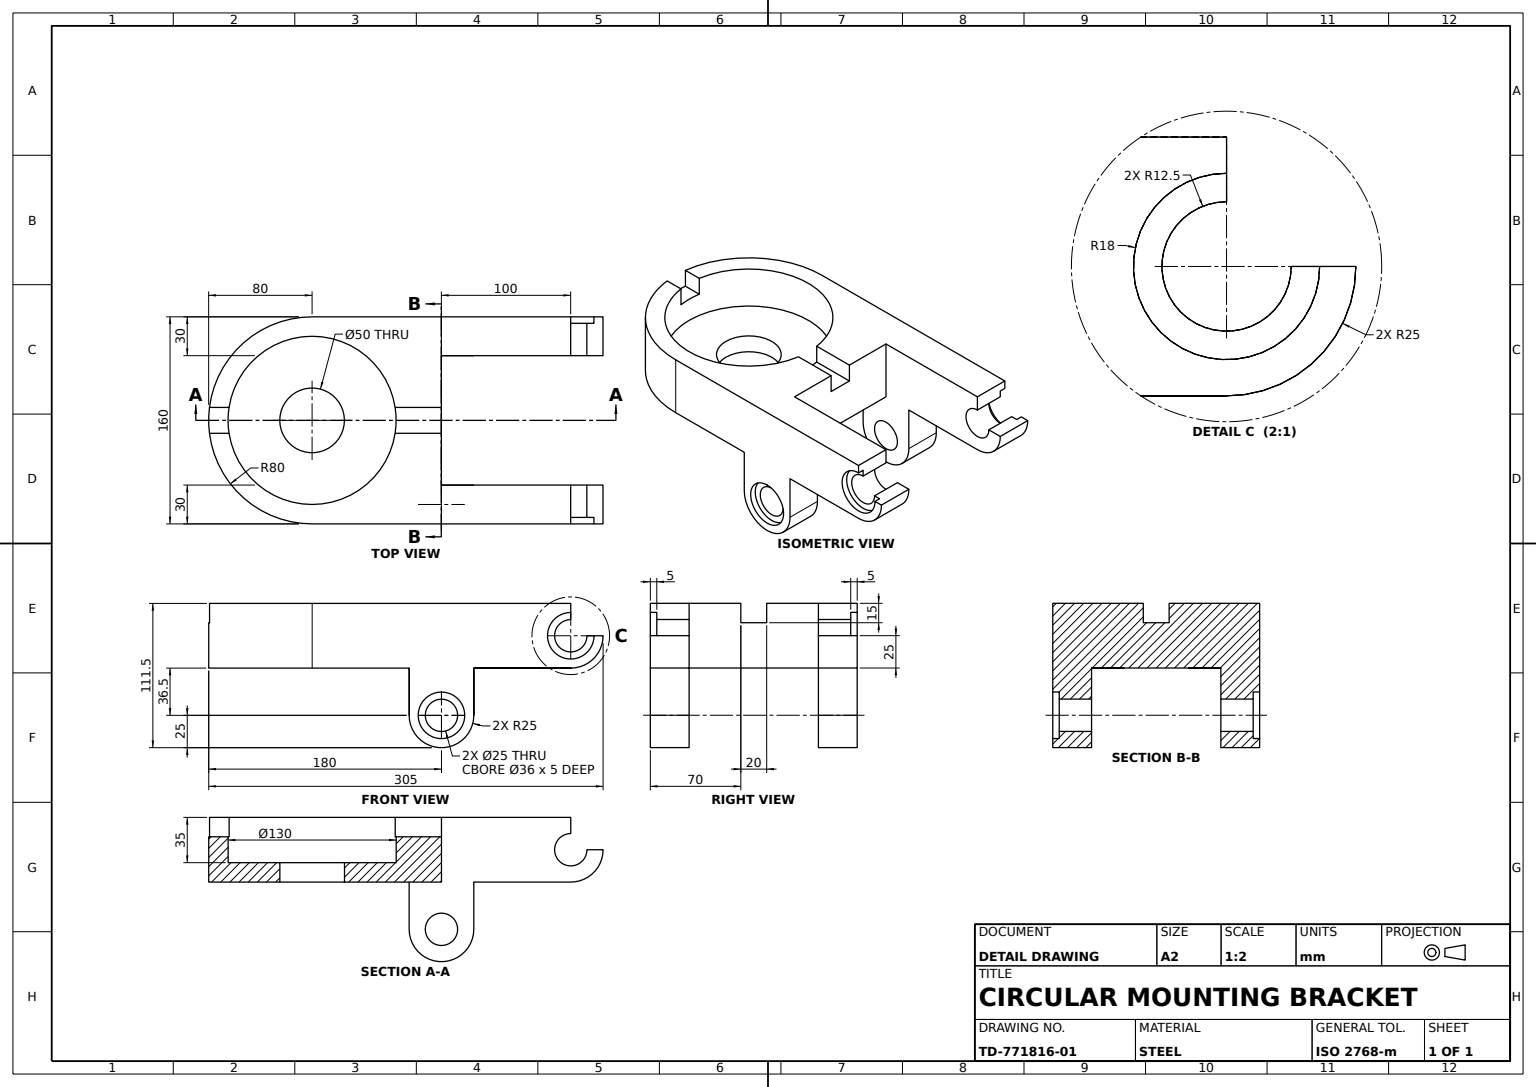
ISO-10303-21;
HEADER;
FILE_DESCRIPTION((''),'2;1');
FILE_NAME('','',(''),(''),'','','');
FILE_SCHEMA(('AUTOMOTIVE_DESIGN'));
ENDSEC;
DATA;
#1=APPLICATION_CONTEXT('');
#2=PRODUCT_CONTEXT('',#1,'mechanical');
#3=PRODUCT('','','',(#2));
#4=PRODUCT_DEFINITION_FORMATION('','',#3);
#5=PRODUCT_DEFINITION_CONTEXT('',#1,'design');
#6=PRODUCT_DEFINITION('','',#4,#5);
#7=PRODUCT_DEFINITION_SHAPE('','',#6);
#8=(LENGTH_UNIT()NAMED_UNIT(*)SI_UNIT(.MILLI.,.METRE.));
#9=(NAMED_UNIT(*)PLANE_ANGLE_UNIT()SI_UNIT($,.RADIAN.));
#10=(NAMED_UNIT(*)SI_UNIT($,.STERADIAN.)SOLID_ANGLE_UNIT());
#11=UNCERTAINTY_MEASURE_WITH_UNIT(LENGTH_MEASURE(0.005),#8,'distance_accuracy_value','');
#12=(GEOMETRIC_REPRESENTATION_CONTEXT(3)GLOBAL_UNCERTAINTY_ASSIGNED_CONTEXT((#11))GLOBAL_UNIT_ASSIGNED_CONTEXT((#8,#9,#10))REPRESENTATION_CONTEXT('',''));
#13=CARTESIAN_POINT('',(212.5,50.,25.));
#14=VERTEX_POINT('',#13);
#15=CARTESIAN_POINT('',(200.,50.,37.5));
#16=VERTEX_POINT('',#15);
#17=CARTESIAN_POINT('',(200.,50.,25.));
#18=DIRECTION('',(0.,1.,0.));
#19=DIRECTION('',(-1.,0.,0.));
#20=AXIS2_PLACEMENT_3D('',#17,#18,#19);
#21=CIRCLE('',#20,12.5);
#22=EDGE_CURVE('',#14,#16,#21,.T.);
#23=ORIENTED_EDGE('',*,*,#22,.F.);
#24=CARTESIAN_POINT('',(212.5,75.,25.));
#25=VERTEX_POINT('',#24);
#26=CARTESIAN_POINT('',(212.5,35.,25.));
#27=DIRECTION('',(0.,-1.,0.));
#28=VECTOR('',#27,1000.);
#29=LINE('',#26,#28);
#30=EDGE_CURVE('',#14,#25,#29,.F.);
#31=ORIENTED_EDGE('',*,*,#30,.T.);
#32=CARTESIAN_POINT('',(200.,75.,37.5));
#33=VERTEX_POINT('',#32);
#34=CARTESIAN_POINT('',(200.,75.,25.));
#35=DIRECTION('',(0.,0.,-1.));
#36=AXIS2_PLACEMENT_3D('',#34,#27,#35);
#37=CIRCLE('',#36,12.5);
#38=EDGE_CURVE('',#25,#33,#37,.F.);
#39=ORIENTED_EDGE('',*,*,#38,.T.);
#40=CARTESIAN_POINT('',(200.,35.,37.5));
#41=LINE('',#40,#28);
#42=EDGE_CURVE('',#33,#16,#41,.T.);
#43=ORIENTED_EDGE('',*,*,#42,.T.);
#44=EDGE_LOOP('',(#23,#31,#39,#43));
#45=FACE_BOUND('',#44,.T.);
#46=CARTESIAN_POINT('',(200.,35.,25.));
#47=AXIS2_PLACEMENT_3D('',#46,#27,#35);
#48=CYLINDRICAL_SURFACE('',#47,12.5);
#49=ADVANCED_FACE('',(#45),#48,.F.);
#50=CARTESIAN_POINT('',(100.,-10.,35.));
#51=VERTEX_POINT('',#50);
#52=CARTESIAN_POINT('',(100.,10.,35.));
#53=VERTEX_POINT('',#52);
#54=CARTESIAN_POINT('',(100.,-50.,35.));
#55=VECTOR('',#18,1000.);
#56=LINE('',#54,#55);
#57=EDGE_CURVE('',#51,#53,#56,.T.);
#58=ORIENTED_EDGE('',*,*,#57,.T.);
#59=CARTESIAN_POINT('',(64.226163,10.,35.));
#60=VERTEX_POINT('',#59);
#61=CARTESIAN_POINT('',(115.961249,10.,35.));
#62=VECTOR('',#19,1000.);
#63=LINE('',#61,#62);
#64=EDGE_CURVE('',#60,#53,#63,.F.);
#65=ORIENTED_EDGE('',*,*,#64,.F.);
#66=CARTESIAN_POINT('',(64.226163,-10.,35.));
#67=VERTEX_POINT('',#66);
#68=CARTESIAN_POINT('',(0.,0.,35.));
#69=DIRECTION('',(0.,0.,1.));
#70=DIRECTION('',(1.,0.,0.));
#71=AXIS2_PLACEMENT_3D('',#68,#69,#70);
#72=CIRCLE('',#71,65.);
#73=EDGE_CURVE('',#60,#67,#72,.F.);
#74=ORIENTED_EDGE('',*,*,#73,.T.);
#75=CARTESIAN_POINT('',(-115.961249,-10.,35.));
#76=VECTOR('',#70,1000.);
#77=LINE('',#75,#76);
#78=EDGE_CURVE('',#51,#67,#77,.F.);
#79=ORIENTED_EDGE('',*,*,#78,.F.);
#80=EDGE_LOOP('',(#58,#65,#74,#79));
#81=FACE_BOUND('',#80,.T.);
#82=PLANE('',#71);
#83=ADVANCED_FACE('',(#81),#82,.T.);
#84=CARTESIAN_POINT('',(200.,-80.,0.));
#85=VERTEX_POINT('',#84);
#86=CARTESIAN_POINT('',(125.,-80.,0.));
#87=VERTEX_POINT('',#86);
#88=CARTESIAN_POINT('',(100.,-80.,0.));
#89=LINE('',#88,#62);
#90=EDGE_CURVE('',#85,#87,#89,.T.);
#91=ORIENTED_EDGE('',*,*,#90,.F.);
#92=CARTESIAN_POINT('',(225.,-80.,25.));
#93=VERTEX_POINT('',#92);
#94=CARTESIAN_POINT('',(200.,-80.,25.));
#95=AXIS2_PLACEMENT_3D('',#94,#27,#70);
#96=CIRCLE('',#95,25.);
#97=EDGE_CURVE('',#85,#93,#96,.T.);
#98=ORIENTED_EDGE('',*,*,#97,.T.);
#99=CARTESIAN_POINT('',(218.,-80.,25.));
#100=VERTEX_POINT('',#99);
#101=CARTESIAN_POINT('',(100.,-80.,25.));
#102=LINE('',#101,#76);
#103=EDGE_CURVE('',#100,#93,#102,.T.);
#104=ORIENTED_EDGE('',*,*,#103,.F.);
#105=CARTESIAN_POINT('',(200.,-80.,43.));
#106=VERTEX_POINT('',#105);
#107=AXIS2_PLACEMENT_3D('',#94,#18,#69);
#108=CIRCLE('',#107,18.);
#109=EDGE_CURVE('',#100,#106,#108,.T.);
#110=ORIENTED_EDGE('',*,*,#109,.T.);
#111=CARTESIAN_POINT('',(200.,-80.,50.));
#112=VERTEX_POINT('',#111);
#113=VECTOR('',#35,1000.);
#114=LINE('',#111,#113);
#115=EDGE_CURVE('',#112,#106,#114,.T.);
#116=ORIENTED_EDGE('',*,*,#115,.F.);
#117=CARTESIAN_POINT('',(0.,-80.,50.));
#118=VERTEX_POINT('',#117);
#119=CARTESIAN_POINT('',(100.,-80.,50.));
#120=LINE('',#119,#62);
#121=EDGE_CURVE('',#112,#118,#120,.T.);
#122=ORIENTED_EDGE('',*,*,#121,.T.);
#123=CARTESIAN_POINT('',(0.,-80.,0.));
#124=VERTEX_POINT('',#123);
#125=LINE('',#117,#113);
#126=EDGE_CURVE('',#118,#124,#125,.T.);
#127=ORIENTED_EDGE('',*,*,#126,.T.);
#128=CARTESIAN_POINT('',(75.,-80.,0.));
#129=VERTEX_POINT('',#128);
#130=EDGE_CURVE('',#129,#124,#89,.T.);
#131=ORIENTED_EDGE('',*,*,#130,.F.);
#132=CARTESIAN_POINT('',(75.,-80.,-36.5));
#133=VERTEX_POINT('',#132);
#134=CARTESIAN_POINT('',(75.,-80.,24.));
#135=LINE('',#134,#113);
#136=EDGE_CURVE('',#129,#133,#135,.T.);
#137=ORIENTED_EDGE('',*,*,#136,.T.);
#138=CARTESIAN_POINT('',(125.,-80.,-36.5));
#139=VERTEX_POINT('',#138);
#140=CARTESIAN_POINT('',(100.,-80.,-36.5));
#141=AXIS2_PLACEMENT_3D('',#140,#27,#70);
#142=CIRCLE('',#141,25.);
#143=EDGE_CURVE('',#133,#139,#142,.T.);
#144=ORIENTED_EDGE('',*,*,#143,.T.);
#145=VECTOR('',#69,1000.);
#146=LINE('',#138,#145);
#147=EDGE_CURVE('',#139,#87,#146,.T.);
#148=ORIENTED_EDGE('',*,*,#147,.T.);
#149=EDGE_LOOP('',(#91,#98,#104,#110,#116,#122,#127,#131,#137,#144,#148));
#150=FACE_BOUND('',#149,.T.);
#151=CARTESIAN_POINT('',(100.,-80.,-18.5));
#152=VERTEX_POINT('',#151);
#153=AXIS2_PLACEMENT_3D('',#140,#18,#69);
#154=CIRCLE('',#153,18.);
#155=EDGE_CURVE('',#152,#152,#154,.T.);
#156=ORIENTED_EDGE('',*,*,#155,.T.);
#157=EDGE_LOOP('',(#156));
#158=FACE_BOUND('',#157,.T.);
#159=AXIS2_PLACEMENT_3D('',#119,#27,#35);
#160=PLANE('',#159);
#161=ADVANCED_FACE('',(#150,#158),#160,.T.);
#162=CARTESIAN_POINT('',(75.,80.,0.));
#163=VERTEX_POINT('',#162);
#164=CARTESIAN_POINT('',(75.,80.,-36.5));
#165=VERTEX_POINT('',#164);
#166=CARTESIAN_POINT('',(75.,80.,24.));
#167=LINE('',#166,#113);
#168=EDGE_CURVE('',#163,#165,#167,.T.);
#169=ORIENTED_EDGE('',*,*,#168,.T.);
#170=CARTESIAN_POINT('',(75.,50.,-36.5));
#171=VERTEX_POINT('',#170);
#172=LINE('',#164,#28);
#173=EDGE_CURVE('',#165,#171,#172,.T.);
#174=ORIENTED_EDGE('',*,*,#173,.T.);
#175=CARTESIAN_POINT('',(75.,50.,0.));
#176=VERTEX_POINT('',#175);
#177=CARTESIAN_POINT('',(75.,50.,24.));
#178=LINE('',#177,#113);
#179=EDGE_CURVE('',#176,#171,#178,.T.);
#180=ORIENTED_EDGE('',*,*,#179,.F.);
#181=CARTESIAN_POINT('',(75.,0.,0.));
#182=LINE('',#181,#55);
#183=EDGE_CURVE('',#176,#163,#182,.T.);
#184=ORIENTED_EDGE('',*,*,#183,.T.);
#185=EDGE_LOOP('',(#169,#174,#180,#184));
#186=FACE_BOUND('',#185,.T.);
#187=AXIS2_PLACEMENT_3D('',#166,#19,#69);
#188=PLANE('',#187);
#189=ADVANCED_FACE('',(#186),#188,.T.);
#190=CARTESIAN_POINT('',(112.5,-50.,-36.5));
#191=VERTEX_POINT('',#190);
#192=CARTESIAN_POINT('',(100.,-50.,-36.5));
#193=AXIS2_PLACEMENT_3D('',#192,#27,#70);
#194=CIRCLE('',#193,12.5);
#195=EDGE_CURVE('',#191,#191,#194,.T.);
#196=ORIENTED_EDGE('',*,*,#195,.T.);
#197=EDGE_LOOP('',(#196));
#198=FACE_BOUND('',#197,.T.);
#199=CARTESIAN_POINT('',(75.,-50.,0.));
#200=VERTEX_POINT('',#199);
#201=CARTESIAN_POINT('',(100.,-50.,0.));
#202=VERTEX_POINT('',#201);
#203=CARTESIAN_POINT('',(0.,-50.,0.));
#204=LINE('',#203,#62);
#205=EDGE_CURVE('',#200,#202,#204,.F.);
#206=ORIENTED_EDGE('',*,*,#205,.T.);
#207=CARTESIAN_POINT('',(100.,-50.,50.));
#208=VERTEX_POINT('',#207);
#209=CARTESIAN_POINT('',(100.,-50.,120.));
#210=LINE('',#209,#113);
#211=EDGE_CURVE('',#202,#208,#210,.F.);
#212=ORIENTED_EDGE('',*,*,#211,.T.);
#213=CARTESIAN_POINT('',(200.,-50.,50.));
#214=VERTEX_POINT('',#213);
#215=CARTESIAN_POINT('',(0.,-50.,50.));
#216=LINE('',#215,#62);
#217=EDGE_CURVE('',#214,#208,#216,.T.);
#218=ORIENTED_EDGE('',*,*,#217,.F.);
#219=CARTESIAN_POINT('',(200.,-50.,37.5));
#220=VERTEX_POINT('',#219);
#221=CARTESIAN_POINT('',(200.,-50.,120.));
#222=LINE('',#221,#113);
#223=EDGE_CURVE('',#214,#220,#222,.T.);
#224=ORIENTED_EDGE('',*,*,#223,.T.);
#225=CARTESIAN_POINT('',(212.5,-50.,25.));
#226=VERTEX_POINT('',#225);
#227=CARTESIAN_POINT('',(200.,-50.,25.));
#228=AXIS2_PLACEMENT_3D('',#227,#27,#70);
#229=CIRCLE('',#228,12.5);
#230=EDGE_CURVE('',#220,#226,#229,.T.);
#231=ORIENTED_EDGE('',*,*,#230,.T.);
#232=CARTESIAN_POINT('',(225.,-50.,25.));
#233=VERTEX_POINT('',#232);
#234=CARTESIAN_POINT('',(220.,-50.,25.));
#235=LINE('',#234,#76);
#236=EDGE_CURVE('',#226,#233,#235,.T.);
#237=ORIENTED_EDGE('',*,*,#236,.T.);
#238=CARTESIAN_POINT('',(200.,-50.,0.));
#239=VERTEX_POINT('',#238);
#240=CIRCLE('',#228,25.);
#241=EDGE_CURVE('',#239,#233,#240,.T.);
#242=ORIENTED_EDGE('',*,*,#241,.F.);
#243=CARTESIAN_POINT('',(125.,-50.,0.));
#244=VERTEX_POINT('',#243);
#245=EDGE_CURVE('',#239,#244,#204,.T.);
#246=ORIENTED_EDGE('',*,*,#245,.T.);
#247=CARTESIAN_POINT('',(125.,-50.,-36.5));
#248=VERTEX_POINT('',#247);
#249=LINE('',#247,#145);
#250=EDGE_CURVE('',#248,#244,#249,.T.);
#251=ORIENTED_EDGE('',*,*,#250,.F.);
#252=CARTESIAN_POINT('',(75.,-50.,-36.5));
#253=VERTEX_POINT('',#252);
#254=CIRCLE('',#193,25.);
#255=EDGE_CURVE('',#253,#248,#254,.T.);
#256=ORIENTED_EDGE('',*,*,#255,.F.);
#257=CARTESIAN_POINT('',(75.,-50.,24.));
#258=LINE('',#257,#113);
#259=EDGE_CURVE('',#200,#253,#258,.T.);
#260=ORIENTED_EDGE('',*,*,#259,.F.);
#261=EDGE_LOOP('',(#206,#212,#218,#224,#231,#237,#242,#246,#251,#256,#260));
#262=FACE_BOUND('',#261,.T.);
#263=CARTESIAN_POINT('',(220.,-50.,120.));
#264=AXIS2_PLACEMENT_3D('',#263,#27,#70);
#265=PLANE('',#264);
#266=ADVANCED_FACE('',(#198,#262),#265,.F.);
#267=CARTESIAN_POINT('',(-79.372539,10.,35.));
#268=VERTEX_POINT('',#267);
#269=CARTESIAN_POINT('',(-64.226163,10.,35.));
#270=VERTEX_POINT('',#269);
#271=EDGE_CURVE('',#268,#270,#63,.F.);
#272=ORIENTED_EDGE('',*,*,#271,.F.);
#273=CARTESIAN_POINT('',(-79.372539,-10.,35.));
#274=VERTEX_POINT('',#273);
#275=CIRCLE('',#71,80.);
#276=EDGE_CURVE('',#274,#268,#275,.F.);
#277=ORIENTED_EDGE('',*,*,#276,.F.);
#278=CARTESIAN_POINT('',(-64.226163,-10.,35.));
#279=VERTEX_POINT('',#278);
#280=EDGE_CURVE('',#279,#274,#77,.F.);
#281=ORIENTED_EDGE('',*,*,#280,.F.);
#282=EDGE_CURVE('',#279,#270,#72,.F.);
#283=ORIENTED_EDGE('',*,*,#282,.T.);
#284=EDGE_LOOP('',(#272,#277,#281,#283));
#285=FACE_BOUND('',#284,.T.);
#286=ADVANCED_FACE('',(#285),#82,.T.);
#287=ORIENTED_EDGE('',*,*,#250,.T.);
#288=CARTESIAN_POINT('',(125.,0.,0.));
#289=LINE('',#288,#55);
#290=EDGE_CURVE('',#87,#244,#289,.T.);
#291=ORIENTED_EDGE('',*,*,#290,.F.);
#292=ORIENTED_EDGE('',*,*,#147,.F.);
#293=LINE('',#138,#55);
#294=EDGE_CURVE('',#139,#248,#293,.T.);
#295=ORIENTED_EDGE('',*,*,#294,.T.);
#296=EDGE_LOOP('',(#287,#291,#292,#295));
#297=FACE_BOUND('',#296,.T.);
#298=AXIS2_PLACEMENT_3D('',#138,#19,#69);
#299=PLANE('',#298);
#300=ADVANCED_FACE('',(#297),#299,.F.);
#301=CARTESIAN_POINT('',(100.,-75.,-24.));
#302=VERTEX_POINT('',#301);
#303=CARTESIAN_POINT('',(100.,-75.,-36.5));
#304=AXIS2_PLACEMENT_3D('',#303,#18,#69);
#305=CIRCLE('',#304,12.5);
#306=EDGE_CURVE('',#302,#302,#305,.F.);
#307=ORIENTED_EDGE('',*,*,#306,.F.);
#308=EDGE_LOOP('',(#307));
#309=FACE_BOUND('',#308,.T.);
#310=CARTESIAN_POINT('',(100.,-75.,-18.5));
#311=VERTEX_POINT('',#310);
#312=CIRCLE('',#304,18.);
#313=EDGE_CURVE('',#311,#311,#312,.F.);
#314=ORIENTED_EDGE('',*,*,#313,.T.);
#315=EDGE_LOOP('',(#314));
#316=FACE_BOUND('',#315,.T.);
#317=PLANE('',#304);
#318=ADVANCED_FACE('',(#309,#316),#317,.F.);
#319=CARTESIAN_POINT('',(-64.226163,10.,50.));
#320=VERTEX_POINT('',#319);
#321=CARTESIAN_POINT('',(-79.372539,10.,50.));
#322=VERTEX_POINT('',#321);
#323=CARTESIAN_POINT('',(0.,10.,50.));
#324=LINE('',#323,#62);
#325=EDGE_CURVE('',#320,#322,#324,.T.);
#326=ORIENTED_EDGE('',*,*,#325,.T.);
#327=LINE('',#321,#113);
#328=EDGE_CURVE('',#268,#322,#327,.F.);
#329=ORIENTED_EDGE('',*,*,#328,.F.);
#330=ORIENTED_EDGE('',*,*,#271,.T.);
#331=LINE('',#319,#113);
#332=EDGE_CURVE('',#270,#320,#331,.F.);
#333=ORIENTED_EDGE('',*,*,#332,.T.);
#334=EDGE_LOOP('',(#326,#329,#330,#333));
#335=FACE_BOUND('',#334,.T.);
#336=CARTESIAN_POINT('',(115.961249,10.,62.));
#337=AXIS2_PLACEMENT_3D('',#336,#27,#70);
#338=PLANE('',#337);
#339=ADVANCED_FACE('',(#335),#338,.T.);
#340=ORIENTED_EDGE('',*,*,#195,.F.);
#341=EDGE_LOOP('',(#340));
#342=FACE_BOUND('',#341,.T.);
#343=ORIENTED_EDGE('',*,*,#306,.T.);
#344=EDGE_LOOP('',(#343));
#345=FACE_BOUND('',#344,.T.);
#346=CARTESIAN_POINT('',(100.,-35.,-36.5));
#347=AXIS2_PLACEMENT_3D('',#346,#18,#69);
#348=CYLINDRICAL_SURFACE('',#347,12.5);
#349=ADVANCED_FACE('',(#342,#345),#348,.F.);
#350=CARTESIAN_POINT('',(200.,-75.,43.));
#351=VERTEX_POINT('',#350);
#352=LINE('',#105,#55);
#353=EDGE_CURVE('',#351,#106,#352,.F.);
#354=ORIENTED_EDGE('',*,*,#353,.T.);
#355=ORIENTED_EDGE('',*,*,#109,.F.);
#356=CARTESIAN_POINT('',(218.,-75.,25.));
#357=VERTEX_POINT('',#356);
#358=LINE('',#99,#55);
#359=EDGE_CURVE('',#100,#357,#358,.T.);
#360=ORIENTED_EDGE('',*,*,#359,.T.);
#361=CARTESIAN_POINT('',(200.,-75.,25.));
#362=AXIS2_PLACEMENT_3D('',#361,#18,#69);
#363=CIRCLE('',#362,18.);
#364=EDGE_CURVE('',#351,#357,#363,.F.);
#365=ORIENTED_EDGE('',*,*,#364,.F.);
#366=EDGE_LOOP('',(#354,#355,#360,#365));
#367=FACE_BOUND('',#366,.T.);
#368=CYLINDRICAL_SURFACE('',#107,18.);
#369=ADVANCED_FACE('',(#367),#368,.F.);
#370=CARTESIAN_POINT('',(212.5,-75.,25.));
#371=VERTEX_POINT('',#370);
#372=LINE('',#361,#62);
#373=EDGE_CURVE('',#357,#371,#372,.T.);
#374=ORIENTED_EDGE('',*,*,#373,.T.);
#375=CARTESIAN_POINT('',(200.,-75.,37.5));
#376=VERTEX_POINT('',#375);
#377=CIRCLE('',#362,12.5);
#378=EDGE_CURVE('',#376,#371,#377,.F.);
#379=ORIENTED_EDGE('',*,*,#378,.F.);
#380=LINE('',#361,#145);
#381=EDGE_CURVE('',#376,#351,#380,.T.);
#382=ORIENTED_EDGE('',*,*,#381,.T.);
#383=ORIENTED_EDGE('',*,*,#364,.T.);
#384=EDGE_LOOP('',(#374,#379,#382,#383));
#385=FACE_BOUND('',#384,.T.);
#386=PLANE('',#362);
#387=ADVANCED_FACE('',(#385),#386,.F.);
#388=CARTESIAN_POINT('',(218.,75.,25.));
#389=VERTEX_POINT('',#388);
#390=LINE('',#34,#76);
#391=EDGE_CURVE('',#25,#389,#390,.T.);
#392=ORIENTED_EDGE('',*,*,#391,.F.);
#393=ORIENTED_EDGE('',*,*,#30,.F.);
#394=CARTESIAN_POINT('',(225.,50.,25.));
#395=VERTEX_POINT('',#394);
#396=CARTESIAN_POINT('',(100.,50.,25.));
#397=LINE('',#396,#62);
#398=EDGE_CURVE('',#395,#14,#397,.T.);
#399=ORIENTED_EDGE('',*,*,#398,.F.);
#400=CARTESIAN_POINT('',(225.,80.,25.));
#401=VERTEX_POINT('',#400);
#402=LINE('',#400,#28);
#403=EDGE_CURVE('',#395,#401,#402,.F.);
#404=ORIENTED_EDGE('',*,*,#403,.T.);
#405=CARTESIAN_POINT('',(218.,80.,25.));
#406=VERTEX_POINT('',#405);
#407=CARTESIAN_POINT('',(0.,80.,25.));
#408=LINE('',#407,#62);
#409=EDGE_CURVE('',#401,#406,#408,.T.);
#410=ORIENTED_EDGE('',*,*,#409,.T.);
#411=LINE('',#405,#28);
#412=EDGE_CURVE('',#389,#406,#411,.F.);
#413=ORIENTED_EDGE('',*,*,#412,.F.);
#414=EDGE_LOOP('',(#392,#393,#399,#404,#410,#413));
#415=FACE_BOUND('',#414,.T.);
#416=CARTESIAN_POINT('',(232.692308,-110.,25.));
#417=AXIS2_PLACEMENT_3D('',#416,#35,#19);
#418=PLANE('',#417);
#419=ADVANCED_FACE('',(#415),#418,.F.);
#420=CARTESIAN_POINT('',(125.,80.,0.));
#421=VERTEX_POINT('',#420);
#422=CARTESIAN_POINT('',(125.,50.,0.));
#423=VERTEX_POINT('',#422);
#424=LINE('',#288,#28);
#425=EDGE_CURVE('',#421,#423,#424,.T.);
#426=ORIENTED_EDGE('',*,*,#425,.T.);
#427=CARTESIAN_POINT('',(125.,50.,-36.5));
#428=VERTEX_POINT('',#427);
#429=LINE('',#427,#145);
#430=EDGE_CURVE('',#428,#423,#429,.T.);
#431=ORIENTED_EDGE('',*,*,#430,.F.);
#432=CARTESIAN_POINT('',(125.,80.,-36.5));
#433=VERTEX_POINT('',#432);
#434=LINE('',#432,#28);
#435=EDGE_CURVE('',#433,#428,#434,.T.);
#436=ORIENTED_EDGE('',*,*,#435,.F.);
#437=LINE('',#432,#145);
#438=EDGE_CURVE('',#433,#421,#437,.T.);
#439=ORIENTED_EDGE('',*,*,#438,.T.);
#440=EDGE_LOOP('',(#426,#431,#436,#439));
#441=FACE_BOUND('',#440,.T.);
#442=AXIS2_PLACEMENT_3D('',#432,#70,#35);
#443=PLANE('',#442);
#444=ADVANCED_FACE('',(#441),#443,.T.);
#445=CARTESIAN_POINT('',(100.,80.,-54.5));
#446=VERTEX_POINT('',#445);
#447=CARTESIAN_POINT('',(100.,80.,-36.5));
#448=AXIS2_PLACEMENT_3D('',#447,#27,#35);
#449=CIRCLE('',#448,18.);
#450=EDGE_CURVE('',#446,#446,#449,.T.);
#451=ORIENTED_EDGE('',*,*,#450,.F.);
#452=EDGE_LOOP('',(#451));
#453=FACE_BOUND('',#452,.T.);
#454=CARTESIAN_POINT('',(100.,75.,-54.5));
#455=VERTEX_POINT('',#454);
#456=CARTESIAN_POINT('',(100.,75.,-36.5));
#457=AXIS2_PLACEMENT_3D('',#456,#27,#35);
#458=CIRCLE('',#457,18.);
#459=EDGE_CURVE('',#455,#455,#458,.F.);
#460=ORIENTED_EDGE('',*,*,#459,.F.);
#461=EDGE_LOOP('',(#460));
#462=FACE_BOUND('',#461,.T.);
#463=CYLINDRICAL_SURFACE('',#448,18.);
#464=ADVANCED_FACE('',(#453,#462),#463,.F.);
#465=ORIENTED_EDGE('',*,*,#328,.T.);
#466=CARTESIAN_POINT('',(0.,80.,50.));
#467=VERTEX_POINT('',#466);
#468=CARTESIAN_POINT('',(0.,0.,50.));
#469=AXIS2_PLACEMENT_3D('',#468,#35,#70);
#470=CIRCLE('',#469,80.);
#471=EDGE_CURVE('',#322,#467,#470,.T.);
#472=ORIENTED_EDGE('',*,*,#471,.T.);
#473=CARTESIAN_POINT('',(0.,80.,0.));
#474=VERTEX_POINT('',#473);
#475=LINE('',#466,#113);
#476=EDGE_CURVE('',#467,#474,#475,.T.);
#477=ORIENTED_EDGE('',*,*,#476,.T.);
#478=CARTESIAN_POINT('',(0.,0.,0.));
#479=AXIS2_PLACEMENT_3D('',#478,#35,#70);
#480=CIRCLE('',#479,80.);
#481=EDGE_CURVE('',#124,#474,#480,.T.);
#482=ORIENTED_EDGE('',*,*,#481,.F.);
#483=ORIENTED_EDGE('',*,*,#126,.F.);
#484=CARTESIAN_POINT('',(-79.372539,-10.,50.));
#485=VERTEX_POINT('',#484);
#486=EDGE_CURVE('',#118,#485,#470,.T.);
#487=ORIENTED_EDGE('',*,*,#486,.T.);
#488=LINE('',#484,#113);
#489=EDGE_CURVE('',#485,#274,#488,.T.);
#490=ORIENTED_EDGE('',*,*,#489,.T.);
#491=ORIENTED_EDGE('',*,*,#276,.T.);
#492=EDGE_LOOP('',(#465,#472,#477,#482,#483,#487,#490,#491));
#493=FACE_BOUND('',#492,.T.);
#494=AXIS2_PLACEMENT_3D('',#468,#35,#19);
#495=CYLINDRICAL_SURFACE('',#494,80.);
#496=ADVANCED_FACE('',(#493),#495,.T.);
#497=CARTESIAN_POINT('',(100.,-10.,50.));
#498=VERTEX_POINT('',#497);
#499=CARTESIAN_POINT('',(100.,-10.,120.));
#500=LINE('',#499,#113);
#501=EDGE_CURVE('',#498,#51,#500,.T.);
#502=ORIENTED_EDGE('',*,*,#501,.T.);
#503=ORIENTED_EDGE('',*,*,#78,.T.);
#504=CARTESIAN_POINT('',(64.226163,-10.,50.));
#505=VERTEX_POINT('',#504);
#506=LINE('',#504,#113);
#507=EDGE_CURVE('',#67,#505,#506,.F.);
#508=ORIENTED_EDGE('',*,*,#507,.T.);
#509=CARTESIAN_POINT('',(0.,-10.,50.));
#510=LINE('',#509,#76);
#511=EDGE_CURVE('',#505,#498,#510,.T.);
#512=ORIENTED_EDGE('',*,*,#511,.T.);
#513=EDGE_LOOP('',(#502,#503,#508,#512));
#514=FACE_BOUND('',#513,.T.);
#515=CARTESIAN_POINT('',(-115.961249,-10.,62.));
#516=AXIS2_PLACEMENT_3D('',#515,#18,#19);
#517=PLANE('',#516);
#518=ADVANCED_FACE('',(#514),#517,.T.);
#519=ORIENTED_EDGE('',*,*,#90,.T.);
#520=ORIENTED_EDGE('',*,*,#290,.T.);
#521=ORIENTED_EDGE('',*,*,#245,.F.);
#522=LINE('',#84,#55);
#523=EDGE_CURVE('',#85,#239,#522,.T.);
#524=ORIENTED_EDGE('',*,*,#523,.F.);
#525=EDGE_LOOP('',(#519,#520,#521,#524));
#526=FACE_BOUND('',#525,.T.);
#527=AXIS2_PLACEMENT_3D('',#478,#35,#19);
#528=PLANE('',#527);
#529=ADVANCED_FACE('',(#526),#528,.T.);
#530=ORIENTED_EDGE('',*,*,#236,.F.);
#531=CARTESIAN_POINT('',(212.5,-35.,25.));
#532=LINE('',#531,#55);
#533=EDGE_CURVE('',#371,#226,#532,.T.);
#534=ORIENTED_EDGE('',*,*,#533,.F.);
#535=ORIENTED_EDGE('',*,*,#373,.F.);
#536=ORIENTED_EDGE('',*,*,#359,.F.);
#537=ORIENTED_EDGE('',*,*,#103,.T.);
#538=LINE('',#92,#55);
#539=EDGE_CURVE('',#233,#93,#538,.F.);
#540=ORIENTED_EDGE('',*,*,#539,.F.);
#541=EDGE_LOOP('',(#530,#534,#535,#536,#537,#540));
#542=FACE_BOUND('',#541,.T.);
#543=ADVANCED_FACE('',(#542),#418,.F.);
#544=CARTESIAN_POINT('',(-65.,0.,15.));
#545=VERTEX_POINT('',#544);
#546=CARTESIAN_POINT('',(0.,0.,15.));
#547=AXIS2_PLACEMENT_3D('',#546,#35,#19);
#548=CIRCLE('',#547,65.);
#549=EDGE_CURVE('',#545,#545,#548,.F.);
#550=ORIENTED_EDGE('',*,*,#549,.F.);
#551=EDGE_LOOP('',(#550));
#552=FACE_BOUND('',#551,.T.);
#553=CARTESIAN_POINT('',(64.226163,10.,50.));
#554=VERTEX_POINT('',#553);
#555=CIRCLE('',#494,65.);
#556=EDGE_CURVE('',#320,#554,#555,.T.);
#557=ORIENTED_EDGE('',*,*,#556,.F.);
#558=ORIENTED_EDGE('',*,*,#332,.F.);
#559=ORIENTED_EDGE('',*,*,#282,.F.);
#560=CARTESIAN_POINT('',(-64.226163,-10.,50.));
#561=VERTEX_POINT('',#560);
#562=LINE('',#560,#113);
#563=EDGE_CURVE('',#561,#279,#562,.T.);
#564=ORIENTED_EDGE('',*,*,#563,.F.);
#565=EDGE_CURVE('',#505,#561,#555,.T.);
#566=ORIENTED_EDGE('',*,*,#565,.F.);
#567=ORIENTED_EDGE('',*,*,#507,.F.);
#568=ORIENTED_EDGE('',*,*,#73,.F.);
#569=LINE('',#553,#113);
#570=EDGE_CURVE('',#554,#60,#569,.T.);
#571=ORIENTED_EDGE('',*,*,#570,.F.);
#572=EDGE_LOOP('',(#557,#558,#559,#564,#566,#567,#568,#571));
#573=FACE_BOUND('',#572,.T.);
#574=CYLINDRICAL_SURFACE('',#494,65.);
#575=ADVANCED_FACE('',(#552,#573),#574,.F.);
#576=CARTESIAN_POINT('',(87.5,50.,-36.5));
#577=VERTEX_POINT('',#576);
#578=CARTESIAN_POINT('',(100.,50.,-36.5));
#579=AXIS2_PLACEMENT_3D('',#578,#18,#19);
#580=CIRCLE('',#579,12.5);
#581=EDGE_CURVE('',#577,#577,#580,.T.);
#582=ORIENTED_EDGE('',*,*,#581,.T.);
#583=EDGE_LOOP('',(#582));
#584=FACE_BOUND('',#583,.T.);
#585=CARTESIAN_POINT('',(100.,50.,50.));
#586=VERTEX_POINT('',#585);
#587=CARTESIAN_POINT('',(200.,50.,50.));
#588=VERTEX_POINT('',#587);
#589=CARTESIAN_POINT('',(0.,50.,50.));
#590=LINE('',#589,#76);
#591=EDGE_CURVE('',#586,#588,#590,.T.);
#592=ORIENTED_EDGE('',*,*,#591,.F.);
#593=CARTESIAN_POINT('',(100.,50.,0.));
#594=VERTEX_POINT('',#593);
#595=CARTESIAN_POINT('',(100.,50.,120.));
#596=LINE('',#595,#113);
#597=EDGE_CURVE('',#594,#586,#596,.F.);
#598=ORIENTED_EDGE('',*,*,#597,.F.);
#599=CARTESIAN_POINT('',(0.,50.,0.));
#600=LINE('',#599,#62);
#601=EDGE_CURVE('',#594,#176,#600,.T.);
#602=ORIENTED_EDGE('',*,*,#601,.T.);
#603=ORIENTED_EDGE('',*,*,#179,.T.);
#604=AXIS2_PLACEMENT_3D('',#578,#27,#70);
#605=CIRCLE('',#604,25.);
#606=EDGE_CURVE('',#171,#428,#605,.T.);
#607=ORIENTED_EDGE('',*,*,#606,.T.);
#608=ORIENTED_EDGE('',*,*,#430,.T.);
#609=CARTESIAN_POINT('',(200.,50.,0.));
#610=VERTEX_POINT('',#609);
#611=LINE('',#599,#76);
#612=EDGE_CURVE('',#423,#610,#611,.T.);
#613=ORIENTED_EDGE('',*,*,#612,.T.);
#614=AXIS2_PLACEMENT_3D('',#17,#27,#70);
#615=CIRCLE('',#614,25.);
#616=EDGE_CURVE('',#610,#395,#615,.T.);
#617=ORIENTED_EDGE('',*,*,#616,.T.);
#618=ORIENTED_EDGE('',*,*,#398,.T.);
#619=ORIENTED_EDGE('',*,*,#22,.T.);
#620=CARTESIAN_POINT('',(200.,50.,120.));
#621=LINE('',#620,#145);
#622=EDGE_CURVE('',#16,#588,#621,.T.);
#623=ORIENTED_EDGE('',*,*,#622,.T.);
#624=EDGE_LOOP('',(#592,#598,#602,#603,#607,#608,#613,#617,#618,#619,#623));
#625=FACE_BOUND('',#624,.T.);
#626=AXIS2_PLACEMENT_3D('',#595,#18,#19);
#627=PLANE('',#626);
#628=ADVANCED_FACE('',(#584,#625),#627,.F.);
#629=ORIENTED_EDGE('',*,*,#435,.T.);
#630=ORIENTED_EDGE('',*,*,#606,.F.);
#631=ORIENTED_EDGE('',*,*,#173,.F.);
#632=AXIS2_PLACEMENT_3D('',#447,#27,#70);
#633=CIRCLE('',#632,25.);
#634=EDGE_CURVE('',#165,#433,#633,.T.);
#635=ORIENTED_EDGE('',*,*,#634,.T.);
#636=EDGE_LOOP('',(#629,#630,#631,#635));
#637=FACE_BOUND('',#636,.T.);
#638=CYLINDRICAL_SURFACE('',#448,25.);
#639=ADVANCED_FACE('',(#637),#638,.T.);
#640=CARTESIAN_POINT('',(-25.,0.,0.));
#641=VERTEX_POINT('',#640);
#642=CIRCLE('',#527,25.);
#643=EDGE_CURVE('',#641,#641,#642,.T.);
#644=ORIENTED_EDGE('',*,*,#643,.F.);
#645=EDGE_LOOP('',(#644));
#646=FACE_BOUND('',#645,.T.);
#647=CARTESIAN_POINT('',(100.,0.,0.));
#648=LINE('',#647,#55);
#649=EDGE_CURVE('',#202,#594,#648,.T.);
#650=ORIENTED_EDGE('',*,*,#649,.F.);
#651=ORIENTED_EDGE('',*,*,#205,.F.);
#652=LINE('',#181,#28);
#653=EDGE_CURVE('',#200,#129,#652,.T.);
#654=ORIENTED_EDGE('',*,*,#653,.T.);
#655=ORIENTED_EDGE('',*,*,#130,.T.);
#656=ORIENTED_EDGE('',*,*,#481,.T.);
#657=LINE('',#473,#76);
#658=EDGE_CURVE('',#474,#163,#657,.T.);
#659=ORIENTED_EDGE('',*,*,#658,.T.);
#660=ORIENTED_EDGE('',*,*,#183,.F.);
#661=ORIENTED_EDGE('',*,*,#601,.F.);
#662=EDGE_LOOP('',(#650,#651,#654,#655,#656,#659,#660,#661));
#663=FACE_BOUND('',#662,.T.);
#664=ADVANCED_FACE('',(#646,#663),#528,.T.);
#665=ORIENTED_EDGE('',*,*,#155,.F.);
#666=EDGE_LOOP('',(#665));
#667=FACE_BOUND('',#666,.T.);
#668=ORIENTED_EDGE('',*,*,#313,.F.);
#669=EDGE_LOOP('',(#668));
#670=FACE_BOUND('',#669,.T.);
#671=CYLINDRICAL_SURFACE('',#153,18.);
#672=ADVANCED_FACE('',(#667,#670),#671,.F.);
#673=CARTESIAN_POINT('',(200.,80.,50.));
#674=VERTEX_POINT('',#673);
#675=LINE('',#111,#55);
#676=EDGE_CURVE('',#588,#674,#675,.T.);
#677=ORIENTED_EDGE('',*,*,#676,.F.);
#678=ORIENTED_EDGE('',*,*,#622,.F.);
#679=ORIENTED_EDGE('',*,*,#42,.F.);
#680=CARTESIAN_POINT('',(200.,75.,43.));
#681=VERTEX_POINT('',#680);
#682=LINE('',#34,#113);
#683=EDGE_CURVE('',#681,#33,#682,.T.);
#684=ORIENTED_EDGE('',*,*,#683,.F.);
#685=CARTESIAN_POINT('',(200.,80.,43.));
#686=VERTEX_POINT('',#685);
#687=LINE('',#685,#28);
#688=EDGE_CURVE('',#686,#681,#687,.T.);
#689=ORIENTED_EDGE('',*,*,#688,.F.);
#690=LINE('',#673,#145);
#691=EDGE_CURVE('',#686,#674,#690,.T.);
#692=ORIENTED_EDGE('',*,*,#691,.T.);
#693=EDGE_LOOP('',(#677,#678,#679,#684,#689,#692));
#694=FACE_BOUND('',#693,.T.);
#695=CARTESIAN_POINT('',(200.,-110.,25.));
#696=AXIS2_PLACEMENT_3D('',#695,#19,#69);
#697=PLANE('',#696);
#698=ADVANCED_FACE('',(#694),#697,.F.);
#699=ORIENTED_EDGE('',*,*,#294,.F.);
#700=ORIENTED_EDGE('',*,*,#143,.F.);
#701=LINE('',#132,#55);
#702=EDGE_CURVE('',#133,#253,#701,.T.);
#703=ORIENTED_EDGE('',*,*,#702,.T.);
#704=ORIENTED_EDGE('',*,*,#255,.T.);
#705=EDGE_LOOP('',(#699,#700,#703,#704));
#706=FACE_BOUND('',#705,.T.);
#707=CYLINDRICAL_SURFACE('',#153,25.);
#708=ADVANCED_FACE('',(#706),#707,.T.);
#709=ORIENTED_EDGE('',*,*,#259,.T.);
#710=ORIENTED_EDGE('',*,*,#702,.F.);
#711=ORIENTED_EDGE('',*,*,#136,.F.);
#712=ORIENTED_EDGE('',*,*,#653,.F.);
#713=EDGE_LOOP('',(#709,#710,#711,#712));
#714=FACE_BOUND('',#713,.T.);
#715=AXIS2_PLACEMENT_3D('',#134,#70,#35);
#716=PLANE('',#715);
#717=ADVANCED_FACE('',(#714),#716,.F.);
#718=CARTESIAN_POINT('',(100.,0.,50.));
#719=LINE('',#718,#55);
#720=EDGE_CURVE('',#208,#498,#719,.T.);
#721=ORIENTED_EDGE('',*,*,#720,.T.);
#722=ORIENTED_EDGE('',*,*,#511,.F.);
#723=ORIENTED_EDGE('',*,*,#565,.T.);
#724=EDGE_CURVE('',#485,#561,#510,.T.);
#725=ORIENTED_EDGE('',*,*,#724,.F.);
#726=ORIENTED_EDGE('',*,*,#486,.F.);
#727=ORIENTED_EDGE('',*,*,#121,.F.);
#728=EDGE_CURVE('',#112,#214,#675,.T.);
#729=ORIENTED_EDGE('',*,*,#728,.T.);
#730=ORIENTED_EDGE('',*,*,#217,.T.);
#731=EDGE_LOOP('',(#721,#722,#723,#725,#726,#727,#729,#730));
#732=FACE_BOUND('',#731,.T.);
#733=PLANE('',#494);
#734=ADVANCED_FACE('',(#732),#733,.F.);
#735=CARTESIAN_POINT('',(100.,10.,50.));
#736=VERTEX_POINT('',#735);
#737=EDGE_CURVE('',#736,#586,#719,.T.);
#738=ORIENTED_EDGE('',*,*,#737,.T.);
#739=ORIENTED_EDGE('',*,*,#591,.T.);
#740=ORIENTED_EDGE('',*,*,#676,.T.);
#741=LINE('',#466,#76);
#742=EDGE_CURVE('',#467,#674,#741,.T.);
#743=ORIENTED_EDGE('',*,*,#742,.F.);
#744=ORIENTED_EDGE('',*,*,#471,.F.);
#745=ORIENTED_EDGE('',*,*,#325,.F.);
#746=ORIENTED_EDGE('',*,*,#556,.T.);
#747=EDGE_CURVE('',#736,#554,#324,.T.);
#748=ORIENTED_EDGE('',*,*,#747,.F.);
#749=EDGE_LOOP('',(#738,#739,#740,#743,#744,#745,#746,#748));
#750=FACE_BOUND('',#749,.T.);
#751=ADVANCED_FACE('',(#750),#733,.F.);
#752=ORIENTED_EDGE('',*,*,#581,.F.);
#753=EDGE_LOOP('',(#752));
#754=FACE_BOUND('',#753,.T.);
#755=CARTESIAN_POINT('',(100.,75.,-49.));
#756=VERTEX_POINT('',#755);
#757=CIRCLE('',#457,12.5);
#758=EDGE_CURVE('',#756,#756,#757,.F.);
#759=ORIENTED_EDGE('',*,*,#758,.T.);
#760=EDGE_LOOP('',(#759));
#761=FACE_BOUND('',#760,.T.);
#762=CARTESIAN_POINT('',(100.,35.,-36.5));
#763=AXIS2_PLACEMENT_3D('',#762,#27,#35);
#764=CYLINDRICAL_SURFACE('',#763,12.5);
#765=ADVANCED_FACE('',(#754,#761),#764,.F.);
#766=ORIENTED_EDGE('',*,*,#724,.T.);
#767=ORIENTED_EDGE('',*,*,#563,.T.);
#768=ORIENTED_EDGE('',*,*,#280,.T.);
#769=ORIENTED_EDGE('',*,*,#489,.F.);
#770=EDGE_LOOP('',(#766,#767,#768,#769));
#771=FACE_BOUND('',#770,.T.);
#772=ADVANCED_FACE('',(#771),#517,.T.);
#773=ORIENTED_EDGE('',*,*,#643,.T.);
#774=EDGE_LOOP('',(#773));
#775=FACE_BOUND('',#774,.T.);
#776=CARTESIAN_POINT('',(-25.,0.,15.));
#777=VERTEX_POINT('',#776);
#778=CIRCLE('',#547,25.);
#779=EDGE_CURVE('',#777,#777,#778,.T.);
#780=ORIENTED_EDGE('',*,*,#779,.F.);
#781=EDGE_LOOP('',(#780));
#782=FACE_BOUND('',#781,.T.);
#783=CYLINDRICAL_SURFACE('',#547,25.);
#784=ADVANCED_FACE('',(#775,#782),#783,.F.);
#785=ORIENTED_EDGE('',*,*,#378,.T.);
#786=ORIENTED_EDGE('',*,*,#533,.T.);
#787=ORIENTED_EDGE('',*,*,#230,.F.);
#788=CARTESIAN_POINT('',(200.,-35.,37.5));
#789=LINE('',#788,#55);
#790=EDGE_CURVE('',#220,#376,#789,.F.);
#791=ORIENTED_EDGE('',*,*,#790,.T.);
#792=EDGE_LOOP('',(#785,#786,#787,#791));
#793=FACE_BOUND('',#792,.T.);
#794=CARTESIAN_POINT('',(200.,-35.,25.));
#795=AXIS2_PLACEMENT_3D('',#794,#18,#69);
#796=CYLINDRICAL_SURFACE('',#795,12.5);
#797=ADVANCED_FACE('',(#793),#796,.F.);
#798=ORIENTED_EDGE('',*,*,#241,.T.);
#799=ORIENTED_EDGE('',*,*,#539,.T.);
#800=ORIENTED_EDGE('',*,*,#97,.F.);
#801=ORIENTED_EDGE('',*,*,#523,.T.);
#802=EDGE_LOOP('',(#798,#799,#800,#801));
#803=FACE_BOUND('',#802,.T.);
#804=CYLINDRICAL_SURFACE('',#107,25.);
#805=ADVANCED_FACE('',(#803),#804,.T.);
#806=CIRCLE('',#36,18.);
#807=EDGE_CURVE('',#389,#681,#806,.F.);
#808=ORIENTED_EDGE('',*,*,#807,.F.);
#809=ORIENTED_EDGE('',*,*,#412,.T.);
#810=CARTESIAN_POINT('',(200.,80.,25.));
#811=AXIS2_PLACEMENT_3D('',#810,#27,#35);
#812=CIRCLE('',#811,18.);
#813=EDGE_CURVE('',#686,#406,#812,.T.);
#814=ORIENTED_EDGE('',*,*,#813,.F.);
#815=ORIENTED_EDGE('',*,*,#688,.T.);
#816=EDGE_LOOP('',(#808,#809,#814,#815));
#817=FACE_BOUND('',#816,.T.);
#818=CYLINDRICAL_SURFACE('',#811,18.);
#819=ADVANCED_FACE('',(#817),#818,.F.);
#820=ORIENTED_EDGE('',*,*,#38,.F.);
#821=ORIENTED_EDGE('',*,*,#391,.T.);
#822=ORIENTED_EDGE('',*,*,#807,.T.);
#823=ORIENTED_EDGE('',*,*,#683,.T.);
#824=EDGE_LOOP('',(#820,#821,#822,#823));
#825=FACE_BOUND('',#824,.T.);
#826=PLANE('',#36);
#827=ADVANCED_FACE('',(#825),#826,.F.);
#828=ORIENTED_EDGE('',*,*,#450,.T.);
#829=EDGE_LOOP('',(#828));
#830=FACE_BOUND('',#829,.T.);
#831=ORIENTED_EDGE('',*,*,#438,.F.);
#832=ORIENTED_EDGE('',*,*,#634,.F.);
#833=ORIENTED_EDGE('',*,*,#168,.F.);
#834=ORIENTED_EDGE('',*,*,#658,.F.);
#835=ORIENTED_EDGE('',*,*,#476,.F.);
#836=ORIENTED_EDGE('',*,*,#742,.T.);
#837=ORIENTED_EDGE('',*,*,#691,.F.);
#838=ORIENTED_EDGE('',*,*,#813,.T.);
#839=ORIENTED_EDGE('',*,*,#409,.F.);
#840=CARTESIAN_POINT('',(200.,80.,0.));
#841=VERTEX_POINT('',#840);
#842=AXIS2_PLACEMENT_3D('',#810,#27,#70);
#843=CIRCLE('',#842,25.);
#844=EDGE_CURVE('',#841,#401,#843,.T.);
#845=ORIENTED_EDGE('',*,*,#844,.F.);
#846=EDGE_CURVE('',#421,#841,#657,.T.);
#847=ORIENTED_EDGE('',*,*,#846,.F.);
#848=EDGE_LOOP('',(#831,#832,#833,#834,#835,#836,#837,#838,#839,#845,#847));
#849=FACE_BOUND('',#848,.T.);
#850=AXIS2_PLACEMENT_3D('',#466,#18,#69);
#851=PLANE('',#850);
#852=ADVANCED_FACE('',(#830,#849),#851,.T.);
#853=ORIENTED_EDGE('',*,*,#758,.F.);
#854=EDGE_LOOP('',(#853));
#855=FACE_BOUND('',#854,.T.);
#856=ORIENTED_EDGE('',*,*,#459,.T.);
#857=EDGE_LOOP('',(#856));
#858=FACE_BOUND('',#857,.T.);
#859=PLANE('',#457);
#860=ADVANCED_FACE('',(#855,#858),#859,.F.);
#861=ORIENTED_EDGE('',*,*,#844,.T.);
#862=ORIENTED_EDGE('',*,*,#403,.F.);
#863=ORIENTED_EDGE('',*,*,#616,.F.);
#864=EDGE_CURVE('',#610,#841,#522,.T.);
#865=ORIENTED_EDGE('',*,*,#864,.T.);
#866=EDGE_LOOP('',(#861,#862,#863,#865));
#867=FACE_BOUND('',#866,.T.);
#868=CYLINDRICAL_SURFACE('',#811,25.);
#869=ADVANCED_FACE('',(#867),#868,.T.);
#870=ORIENTED_EDGE('',*,*,#846,.T.);
#871=ORIENTED_EDGE('',*,*,#864,.F.);
#872=ORIENTED_EDGE('',*,*,#612,.F.);
#873=ORIENTED_EDGE('',*,*,#425,.F.);
#874=EDGE_LOOP('',(#870,#871,#872,#873));
#875=FACE_BOUND('',#874,.T.);
#876=ADVANCED_FACE('',(#875),#528,.T.);
#877=CARTESIAN_POINT('',(100.,10.,120.));
#878=LINE('',#877,#145);
#879=EDGE_CURVE('',#53,#736,#878,.T.);
#880=ORIENTED_EDGE('',*,*,#879,.F.);
#881=ORIENTED_EDGE('',*,*,#57,.F.);
#882=ORIENTED_EDGE('',*,*,#501,.F.);
#883=ORIENTED_EDGE('',*,*,#720,.F.);
#884=ORIENTED_EDGE('',*,*,#211,.F.);
#885=ORIENTED_EDGE('',*,*,#649,.T.);
#886=ORIENTED_EDGE('',*,*,#597,.T.);
#887=ORIENTED_EDGE('',*,*,#737,.F.);
#888=EDGE_LOOP('',(#880,#881,#882,#883,#884,#885,#886,#887));
#889=FACE_BOUND('',#888,.T.);
#890=AXIS2_PLACEMENT_3D('',#209,#19,#69);
#891=PLANE('',#890);
#892=ADVANCED_FACE('',(#889),#891,.F.);
#893=ORIENTED_EDGE('',*,*,#728,.F.);
#894=ORIENTED_EDGE('',*,*,#115,.T.);
#895=ORIENTED_EDGE('',*,*,#353,.F.);
#896=ORIENTED_EDGE('',*,*,#381,.F.);
#897=ORIENTED_EDGE('',*,*,#790,.F.);
#898=ORIENTED_EDGE('',*,*,#223,.F.);
#899=EDGE_LOOP('',(#893,#894,#895,#896,#897,#898));
#900=FACE_BOUND('',#899,.T.);
#901=ADVANCED_FACE('',(#900),#697,.F.);
#902=ORIENTED_EDGE('',*,*,#64,.T.);
#903=ORIENTED_EDGE('',*,*,#879,.T.);
#904=ORIENTED_EDGE('',*,*,#747,.T.);
#905=ORIENTED_EDGE('',*,*,#570,.T.);
#906=EDGE_LOOP('',(#902,#903,#904,#905));
#907=FACE_BOUND('',#906,.T.);
#908=ADVANCED_FACE('',(#907),#338,.T.);
#909=ORIENTED_EDGE('',*,*,#779,.T.);
#910=EDGE_LOOP('',(#909));
#911=FACE_BOUND('',#910,.T.);
#912=ORIENTED_EDGE('',*,*,#549,.T.);
#913=EDGE_LOOP('',(#912));
#914=FACE_BOUND('',#913,.T.);
#915=PLANE('',#547);
#916=ADVANCED_FACE('',(#911,#914),#915,.F.);
#917=CLOSED_SHELL('',(#49,#83,#161,#189,#266,#286,#300,#318,#339,#349,#369,#387,#419,#444,#464,#496,#518,#529,#543,#575,#628,#639,#664,#672,#698,#708,#717,#734,#751,#765,#772,#784,#797,#805,#819,#827,#852,#860,#869,#876,#892,#901,#908,#916));
#918=MANIFOLD_SOLID_BREP('',#917);
#919=ADVANCED_BREP_SHAPE_REPRESENTATION('',(#918),#12);
#920=SHAPE_DEFINITION_REPRESENTATION(#7,#919);
ENDSEC;
END-ISO-10303-21;
